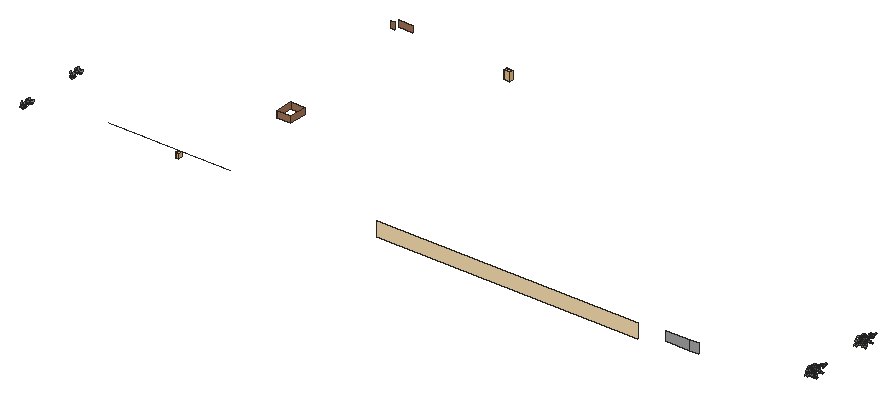
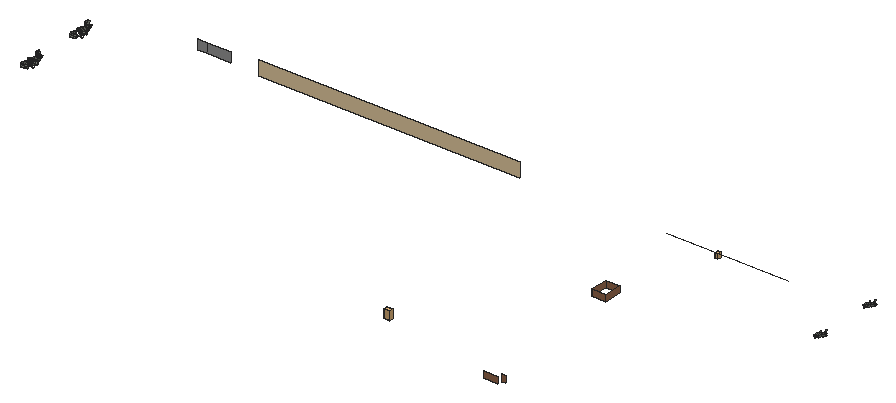
# SketchUp Ruby script. Lengths in inches.
U = 1.inch
M = Sketchup.active_model
def pt(a) = Geom::Point3d.new(a.map { |v| v * U })
def face(e, loops, mat)
  f = e.add_face(loops[0].map { |a| pt(a) })
  loops[1..].each { |l| e.add_face(l.map { |a| pt(a) }).erase! }
  f.material = f.back_material = mat if mat
  f
end
# faces: each face lists its corners as indices into pts; further lists are holes
def faces(e, pts, list, mat = nil) = list.each { |f| face(e, (f[0].is_a?(Array) ? f : [f]).map { |l| l.map { |i| pts[i] } }, mat) }
# xy, xz, yz: faces in a plane at the given z, y or x. An outline is a flat list of corners, or four numbers for a rectangle; further outlines are holes
def ring(l) = l.size == 4 ? [[l[0], l[1]], [l[2], l[1]], [l[2], l[3]], [l[0], l[3]]] : l.each_slice(2).to_a
def flat(e, list, mat, &to3) = list.each { |f| face(e, (f[0].is_a?(Array) ? f : [f]).map { |l| ring(l).map { |u, v| to3.(u, v) } }, mat) }
def xy(e, z, list, mat = nil) = flat(e, list, mat) { |x, y| [x, y, z] }
def xz(e, y, list, mat = nil) = flat(e, list, mat) { |x, z| [x, y, z] }
def yz(e, x, list, mat = nil) = flat(e, list, mat) { |y, z| [x, y, z] }
def lines(e, pts, list) = list.each { |a, b| e.add_line(pt(pts[a]), pt(pts[b])) }
# prism: a flat outline (further loops are holes) pulled along v
def prism(e, loops, v, mat = nil)
  f = face(e, loops, mat); d = Geom::Vector3d.new(v.map { |x| x * U })
  f.pushpull(f.normal.samedirection?(d) ? d.length : -d.length)
end
def box(e, o, s, mat = nil) = prism(e, [[o, [o[0] + s[0], o[1], o[2]], [o[0] + s[0], o[1] + s[1], o[2]], [o[0], o[1] + s[1], o[2]]]], [0, 0, s[2]], mat)
def at(x, y, z, deg = 0) = Geom::Transformation.translation(pt([x, y, z])) * Geom::Transformation.rotation(ORIGIN, Z_AXIS, deg.degrees)
def axes(o, x, y, z) = Geom::Transformation.new([*x, 0, *y, 0, *z, 0, *pt(o).to_a, 1])
def part(name) = M.definitions.add(name)
# library, detail: a bought-in or finely detailed component or shape, given as its bounding box
def library(name, o, s) = part(name).tap { |d| box(d.entities, o, s) }
def detail(e, o, s) = box(e.add_group.entities, o, s)
def put(e, d, t, mat = nil) = e.add_instance(d, t).tap { |i| i.material = mat if mat }
def group(e, t, mat = nil) = e.add_group.tap { |g| g.transformation = t; g.material = mat if mat }.entities
root = M.entities
M.materials.add("Material \#1").color = [140, 140, 140]
M.materials.add("[0032_Moccasin]").color = [255, 228, 181]
M.materials.add("[0132_LightGray]").color = [169, 169, 169]
M.materials.add("[Tile Ceramic Multi]").color = [165, 115, 84]
M.materials.add("viburnumblaasdfas0df1w06d").color = [98, 102, 84]
M.materials.add("viburnumbladsadfasdfad0w122").color = [125, 129, 119]
c1 = part("Component\#315")
p = [[0.25,0,0],[2.05,0.01,0.35],[1.81,4.2,1.66],[0,4.19,1.3125]]
faces(c1.entities,p,[[0,1,2,3]],"viburnumbladsadfasdfad0w122")
c2 = part("viburnumblad2")
put(c2.entities,c1,axes([-19.23,-4.49,-32.18],[83.35428,0,0],[0,79.38502,0],[0,0,83.35428]))
c3 = library("Lamp Wall Outdoor 94-02",[-1.89,-4.65,-3.17],[3.78,4.65,6.35])
c4 = library("3DGeom~3_Defintion",[-83.33,-500,-350],[620.1,1000,533.33])
c5 = part("Component\#314")
p = [[0.14,0,0],[2.58,0.05,0.25],[2.44,5.11,2.64],[0,5.05,2.39]]
faces(c5.entities,p,[[0,1,2,3]],"viburnumblaasdfas0df1w06d")
c6 = part("viburnumblad1\#2")
put(c6.entities,c5,axes([-37.25,6.23,19.31],[75.98784,0,0],[0,65.50676,0],[0,0,75.98784]))
xz(root,218.9375,[[1678.9375,30,2004.71,47.68]],"[0032_Moccasin]")
xz(root,223.9375,[[2036.3125,36,2065.6875,48]],"[0132_LightGray]")
xz(root,340.22,[[1457.08,32,1474.64,40]],"[Tile Ceramic Multi]")
xz(root,362.07,[[1457.08,32,1474.64,40]],"[Tile Ceramic Multi]")
xz(root,529.35,[[1590.92,39.28,1590.76,39.29,1590.92,39.29],[1590.92,39.28,1590.92,39.29,1591.07,39.31],[1590.92,39.28,1591.07,39.31,1591.08,39.29],[1590.76,39.29,1590.62,39.33,1590.77,39.31],[1590.76,39.29,1590.77,39.31,1590.92,39.29],
  [1591.08,39.29,1591.07,39.31,1591.22,39.34],[1591.08,39.29,1591.22,39.34,1591.23,39.33],[1590.77,39.31,1590.62,39.33,1590.62,39.34],[1590.62,39.33,1590.48,39.39,1590.62,39.34],[1591.23,39.33,1591.22,39.34,1591.35,39.4],
  [1591.23,39.33,1591.35,39.4,1591.36,39.39],[1590.62,39.34,1590.48,39.39,1590.49,39.4],[1590.48,39.39,1590.36,39.46,1590.49,39.4],[1591.36,39.39,1591.35,39.4,1591.47,39.47],[1591.36,39.39,1591.47,39.47,1591.48,39.46],
  [1590.49,39.4,1590.36,39.46,1590.37,39.47],[1590.36,39.46,1590.25,39.56,1590.37,39.47],[1591.48,39.46,1591.47,39.47,1591.58,39.57],[1591.48,39.46,1591.58,39.57,1591.59,39.56],[1590.37,39.47,1590.25,39.56,1590.26,39.57],
  [1590.87,39.49,1590.82,39.5,1590.87,39.51],[1590.87,39.49,1590.87,39.51,1590.92,39.5],[1590.87,39.49,1590.92,39.5,1590.92,39.49],[1590.92,39.49,1590.92,39.5,1590.97,39.51],[1590.92,39.49,1590.97,39.51,1590.97,39.49],
  [1590.97,39.49,1590.97,39.51,1591.02,39.52],[1590.97,39.49,1591.02,39.52,1591.02,39.5],[1590.82,39.5,1590.77,39.52,1590.82,39.52],[1590.82,39.5,1590.82,39.52,1590.87,39.51],[1591.02,39.5,1591.02,39.52,1591.06,39.54],
  [1591.02,39.5,1591.06,39.54,1591.07,39.52],[1590.77,39.52,1590.73,39.55,1590.78,39.54],[1590.77,39.52,1590.78,39.54,1590.82,39.52],[1591.07,39.52,1591.06,39.54,1591.1,39.56],[1591.07,39.52,1591.1,39.56,1591.11,39.55]],"Material \#1")
xz(root,531.36,[[1590.92,39.28,1590.92,39.29,1590.76,39.29],[1590.92,39.28,1591.07,39.31,1590.92,39.29],[1590.92,39.28,1591.08,39.29,1591.07,39.31],[1590.76,39.29,1590.77,39.31,1590.62,39.33],[1590.76,39.29,1590.92,39.29,1590.77,39.31],
  [1591.08,39.29,1591.22,39.34,1591.07,39.31],[1591.08,39.29,1591.23,39.33,1591.22,39.34],[1590.77,39.31,1590.62,39.34,1590.62,39.33],[1590.62,39.33,1590.62,39.34,1590.48,39.39],[1591.23,39.33,1591.35,39.4,1591.22,39.34],
  [1591.23,39.33,1591.36,39.39,1591.35,39.4],[1590.62,39.34,1590.49,39.4,1590.48,39.39],[1590.48,39.39,1590.49,39.4,1590.36,39.46],[1591.36,39.39,1591.47,39.47,1591.35,39.4],[1591.36,39.39,1591.48,39.46,1591.47,39.47],
  [1590.49,39.4,1590.37,39.47,1590.36,39.46],[1590.36,39.46,1590.37,39.47,1590.25,39.56],[1591.48,39.46,1591.58,39.57,1591.47,39.47],[1591.48,39.46,1591.59,39.56,1591.58,39.57],[1590.37,39.47,1590.26,39.57,1590.25,39.56],
  [1590.87,39.49,1590.87,39.51,1590.82,39.5],[1590.87,39.49,1590.92,39.49,1590.92,39.5],[1590.87,39.49,1590.92,39.5,1590.87,39.51],[1590.92,39.49,1590.97,39.49,1590.97,39.51],[1590.92,39.49,1590.97,39.51,1590.92,39.5],
  [1590.97,39.49,1591.02,39.5,1591.02,39.52],[1590.97,39.49,1591.02,39.52,1590.97,39.51],[1590.82,39.5,1590.82,39.52,1590.77,39.52],[1590.82,39.5,1590.87,39.51,1590.82,39.52],[1591.02,39.5,1591.06,39.54,1591.02,39.52],
  [1591.02,39.5,1591.07,39.52,1591.06,39.54],[1590.77,39.52,1590.78,39.54,1590.73,39.55],[1590.77,39.52,1590.82,39.52,1590.78,39.54]],"Material \#1")
xz(root,549.6875,[[1431.3125,32,1437.22,40]],"[Tile Ceramic Multi]")
xz(root,555,[[1437.22,32,1454.9375,40]],"[Tile Ceramic Multi]")
yz(root,1457.08,[[340.22,32,362.07,40]],"[Tile Ceramic Multi]")
yz(root,1474.64,[[340.22,32,362.07,40]],"[Tile Ceramic Multi]")
p = [[2065.6875,223.9375,48],[2065.6875,223.9375,36],[2076.625,224.21,36],[2076.625,224.21,48],[1491.42,223.9375,36],[1338.625,223.9375,36]]
faces(root,p,[[0,1,2,3]],"[0132_LightGray]")
lines(root,p,[[4,5]])
put(root,c2,axes([1246.61,280.32,31.73],[0.00136,-0.01101,-0.00167],[0.00866,0.00241,-0.00886],[0.00838,-0.00019,0.00814]))
put(root,c2,axes([1246.61,203.43,31.73],[0.00136,-0.01101,-0.00167],[0.00866,0.00241,-0.00886],[0.00838,-0.00019,0.00814]))
put(root,c2,axes([1248.83,286.96,33.1875],[0.0051,0.01038,-0.00415],[-0.00633,0.00571,0.00604],[0.00802,-0.00053,0.00751]))
put(root,c2,axes([1248.83,210.08,33.1875],[0.0051,0.01038,-0.00415],[-0.00633,0.00571,0.00604],[0.00802,-0.00053,0.00751]))
put(root,c2,axes([1249.1,278.54,33.3],[-0.00142,0.01147,0.00174],[-0.00575,-0.00222,0.00993],[0.01007,0.00035,0.00591]))
put(root,c2,axes([1249.1,201.66,33.3],[-0.00142,0.01147,0.00174],[-0.00575,-0.00222,0.00993],[0.01007,0.00035,0.00591]))
put(root,c2,axes([1247.41,280.15,33.05],[0.00591,-0.00652,-0.00769],[0.005,0.00963,-0.00433],[0.00875,-0.0011,0.00766]))
put(root,c2,axes([1247.41,203.27,33.05],[0.00591,-0.00652,-0.00769],[0.005,0.00963,-0.00433],[0.00875,-0.0011,0.00766]))
put(root,c2,axes([1249.99,287.16,32.28],[-0.00764,0.00611,0.00552],[-0.0043,-0.01063,0.00535],[0.00765,0.00146,0.00773]))
put(root,c2,axes([1249.99,210.27,32.28],[-0.00764,0.00611,0.00552],[-0.0043,-0.01063,0.00535],[0.00765,0.00146,0.00773]))
put(root,c2,axes([1250.43,286.67,33.61],[-0.00217,0.01153,0.00126],[-0.00855,-0.00261,0.00823],[0.00816,0.00055,0.00738]))
put(root,c2,axes([1250.43,209.78,33.61],[-0.00217,0.01153,0.00126],[-0.00855,-0.00261,0.00823],[0.00816,0.00055,0.00738]))
put(root,c2,axes([1248.45,279.5625,34.14],[0.00693,0.00224,-0.00913],[-0.00028,0.01139,0.00259],[0.0094,-0.00132,0.00681]))
put(root,c2,axes([1248.45,202.68,34.14],[0.00693,0.00224,-0.00913],[-0.00028,0.01139,0.00259],[0.0094,-0.00132,0.00681]))
put(root,c2,axes([1248.19,280.29,31.99],[-0.0039,-0.00969,0.00523],[0.00734,-0.00679,-0.00711],[0.00851,0.00087,0.00796]))
put(root,c2,axes([1248.19,203.41,31.99],[-0.0039,-0.00969,0.00523],[0.00734,-0.00679,-0.00711],[0.00851,0.00087,0.00796]))
put(root,c2,axes([1249.72,279.61,32.48],[-0.00693,-0.00224,0.00913],[0.00254,-0.01137,-0.00086],[0.00905,0.00148,0.00724]))
put(root,c2,axes([1249.72,202.73,32.48],[-0.00693,-0.00224,0.00913],[0.00254,-0.01137,-0.00086],[0.00905,0.00148,0.00724]))
put(root,c2,axes([1249.4375,287.32,34.32],[0.00908,0.00254,-0.00688],[-0.00118,0.01053,0.00207],[0.00732,-0.00116,0.00806]))
put(root,c2,axes([1249.4375,210.4375,34.32],[0.00908,0.00254,-0.00688],[-0.00118,0.01053,0.00207],[0.00732,-0.00116,0.00806]))
put(root,c2,axes([1250.64,286.79,35.2],[0.00489,0.00995,-0.00397],[-0.00703,0.00634,0.00672],[0.00802,-0.00053,0.00751]))
put(root,c2,axes([1250.64,209.91,35.2],[0.00489,0.00995,-0.00397],[-0.00703,0.00634,0.00672],[0.00802,-0.00053,0.00751]))
put(root,c2,axes([1248.78,288.22,33.3],[0.00664,-0.00572,-0.00612],[0.00571,0.0099,-0.00294],[0.00728,-0.00165,0.00803]))
put(root,c2,axes([1248.78,211.34,33.3],[0.00664,-0.00572,-0.00612],[0.00571,0.0099,-0.00294],[0.00728,-0.00165,0.00803]))
put(root,c2,axes([1249.06,280.63,33.33],[0.00142,-0.01147,-0.00174],[0.00801,0.00224,-0.0082],[0.00838,-0.00019,0.00814]))
put(root,c2,axes([1249.06,203.75,33.33],[0.00142,-0.01147,-0.00174],[0.00801,0.00224,-0.0082],[0.00838,-0.00019,0.00814]))
put(root,c2,axes([1251.82,286.86,34.32],[-0.00796,0.00636,0.00575],[-0.00398,-0.00984,0.00495],[0.00765,0.00146,0.00773]))
put(root,c2,axes([1251.82,209.98,34.32],[-0.00796,0.00636,0.00575],[-0.00398,-0.00984,0.00495],[0.00765,0.00146,0.00773]))
put(root,c2,axes([1251.07,287.73,33.13],[-0.00908,-0.00254,0.00688],[0.00302,-0.01141,-0.00024],[0.00679,0.00165,0.00837]))
put(root,c2,axes([1251.07,210.84,33.13],[-0.00908,-0.00254,0.00688],[0.00302,-0.01141,-0.00024],[0.00679,0.00165,0.00837]))
put(root,c2,axes([1250.15,288.72,33.78],[0.00217,-0.01153,-0.00126],[0.00998,0.00257,-0.00587],[0.00594,-0.00007,0.00905]))
put(root,c2,axes([1250.15,211.84,33.78],[0.00217,-0.01153,-0.00126],[0.00998,0.00257,-0.00587],[0.00594,-0.00007,0.00905]))
put(root,c2,axes([1250.57,288.28,35.21],[0.00796,-0.00636,-0.00575],[0.00571,0.0099,-0.00294],[0.00646,-0.00097,0.0087]))
put(root,c2,axes([1250.57,211.4,35.21],[0.00796,-0.00636,-0.00575],[0.00571,0.0099,-0.00294],[0.00646,-0.00097,0.0087]))
put(root,c2,axes([1251.75,288.35,34.33],[-0.00489,-0.00995,0.00397],[0.00876,-0.00628,-0.0047],[0.00608,0.00102,0.00892]))
put(root,c2,axes([1251.75,211.47,34.33],[-0.00489,-0.00995,0.00397],[0.00876,-0.00628,-0.0047],[0.00608,0.00102,0.00892]))
put(root,c3,at(1428.92,223.9375,32.6))
put(root,c4,axes([1590.92,531.05,44.51],[0.012,0,0],[0,0,0.01068],[0,0.00833,0]),"Material \#1")
put(root,c2,axes([2183.65,344.92,39.97],[-0.00351,0.01047,-0.00368],[-0.0097,-0.00494,-0.00456],[-0.00545,0.00224,0.00858]))
put(root,c2,axes([2183.65,268.04,39.97],[-0.00351,0.01047,-0.00368],[-0.0097,-0.00494,-0.00456],[-0.00545,0.00224,0.00858]))
put(root,c2,axes([2182.64,345.63,39.1875],[0.00896,0.00518,0.00557],[-0.00429,0.01059,-0.00268],[-0.00611,0.00033,0.00835]))
put(root,c2,axes([2182.64,268.75,39.1875],[0.00896,0.00518,0.00557],[-0.00429,0.01059,-0.00268],[-0.00611,0.00033,0.00835]))
put(root,c2,axes([2183.85,344.63,38.53],[0.00385,0.01107,0.00134],[-0.00965,0.00395,-0.00558],[-0.00546,0.00115,0.0087]))
put(root,c2,axes([2183.85,267.75,38.53],[0.00385,0.01107,0.00134],[-0.00965,0.00395,-0.00558],[-0.00546,0.00115,0.0087]))
put(root,c2,axes([2185.31,344.47,38.125],[-0.00267,0.00936,-0.00422],[-0.0097,-0.00494,-0.00456],[-0.00579,0.00336,0.00814]))
put(root,c2,axes([2185.31,267.59,38.125],[-0.00267,0.00936,-0.00422],[-0.0097,-0.00494,-0.00456],[-0.00579,0.00336,0.00814]))
put(root,c2,axes([2185.14,345.36,39.29],[-0.00882,0.00375,-0.00654],[-0.00425,-0.0099,-0.00033],[-0.00607,0.00296,0.00807]))
put(root,c2,axes([2185.14,268.48,39.29],[-0.00882,0.00375,-0.00654],[-0.00425,-0.0099,-0.00033],[-0.00607,0.00296,0.00807]))
put(root,c2,axes([2184.32,346.22,40.28],[-0.00896,-0.00518,-0.00557],[0.00268,-0.0102,0.00462],[-0.00697,0.00288,0.00746]))
put(root,c2,axes([2184.32,269.34,40.28],[-0.00896,-0.00518,-0.00557],[0.00268,-0.0102,0.00462],[-0.00697,0.00288,0.00746]))
put(root,c2,axes([2183.58,346.0625,38.17],[0.00882,-0.00375,0.00654],[0.00302,0.01118,0.0023],[-0.00701,0.00026,0.00774]))
put(root,c2,axes([2183.58,269.18,38.17],[0.00882,-0.00375,0.00654],[0.00302,0.01118,0.0023],[-0.00701,0.00026,0.00774]))
put(root,c2,axes([2183.31,346.93,39.49],[0.00351,-0.01047,0.00368],[0.00809,0.00534,0.0065],[-0.00763,0.00098,0.00722]))
put(root,c2,axes([2183.31,270.04,39.49],[0.00351,-0.01047,0.00368],[0.00809,0.00534,0.0065],[-0.00763,0.00098,0.00722]))
put(root,c2,axes([2185.88,345.59,38.29],[-0.00935,-0.0054,-0.00582],[0.00241,-0.00918,0.00416],[-0.00697,0.00288,0.00746]))
put(root,c2,axes([2185.88,268.71,38.29],[-0.00935,-0.0054,-0.00582],[0.00241,-0.00918,0.00416],[-0.00697,0.00288,0.00746]))
put(root,c2,axes([2184.64,346.54,38.82],[-0.00385,-0.01107,-0.00134],[0.00835,-0.0037,0.00784],[-0.00761,0.00206,0.00711]))
put(root,c2,axes([2184.64,269.66,38.82],[-0.00385,-0.01107,-0.00134],[0.00835,-0.0037,0.00784],[-0.00761,0.00206,0.00711]))
put(root,c2,axes([2187.57,333.39,39.18],[0.00449,0.0055,0.01006],[-0.01013,0.00737,0.00027],[-0.00579,-0.00855,0.00654]))
put(root,c2,axes([2187.57,256.51,39.18],[0.00449,0.0055,0.01006],[-0.01013,0.00737,0.00027],[-0.00579,-0.00855,0.00654]))
put(root,c2,axes([2184.83,346.18,37.45],[0.00337,-0.01006,0.00353],[0.00874,0.00576,0.00702],[-0.00763,0.00098,0.00722]))
put(root,c2,axes([2184.83,269.3,37.45],[0.00337,-0.01006,0.00353],[0.00874,0.00576,0.00702],[-0.00763,0.00098,0.00722]))
put(root,c2,axes([2188.24,356.2,38.47],[-0.00103,0.00921,-0.00523],[-0.01005,-0.00269,-0.00267],[-0.00353,0.00478,0.00792]))
put(root,c2,axes([2188.24,279.32,38.47],[-0.00103,0.00921,-0.00523],[-0.01005,-0.00269,-0.00267],[-0.00353,0.00478,0.00792]))
put(root,c6,axes([2189.82,342.8,33.29],[-0.00628,0.01217,-0.00276],[-0.013,-0.00799,-0.00559],[-0.00514,0.00045,0.01101]))
put(root,c6,axes([2189.82,265.92,33.29],[-0.00628,0.01217,-0.00276],[-0.013,-0.00799,-0.00559],[-0.00514,0.00045,0.01101]))
put(root,c2,axes([2189.24,333.99,38.72],[-0.00344,0.0098,0.00674],[-0.01109,0.00113,-0.00697],[-0.00574,-0.00778,0.00739]))
put(root,c2,axes([2189.24,257.11,38.72],[-0.00344,0.0098,0.00674],[-0.01109,0.00113,-0.00697],[-0.00574,-0.00778,0.00739]))
put(root,c2,axes([2188.86,332.93,39.97],[-0.00935,0.00836,-0.00053],[-0.00531,-0.00639,-0.00919],[-0.00638,-0.00686,0.0077]))
put(root,c2,axes([2188.86,256.05,39.97],[-0.00935,0.00836,-0.00053],[-0.00531,-0.00639,-0.00919],[-0.00638,-0.00686,0.0077]))
put(root,c2,axes([2188.23,355.64,37.17],[0.00602,0.00882,-0.00114],[-0.00807,0.00476,-0.00535],[-0.00378,0.00387,0.00824]))
put(root,c2,axes([2188.23,278.76,37.17],[0.00602,0.00882,-0.00114],[-0.00807,0.00476,-0.00535],[-0.00378,0.00387,0.00824]))
put(root,c6,axes([2187.39,345.72,36.11],[-0.0079,-0.01009,-0.00146],[0.00852,-0.00752,0.00905],[-0.00687,0.00486,0.00819]))
put(root,c6,axes([2187.39,268.84,36.11],[-0.0079,-0.01009,-0.00146],[0.00852,-0.00752,0.00905],[-0.00687,0.00486,0.00819]))
put(root,c2,axes([2189.43,355.08,36.73],[-0.00059,0.00795,-0.00557],[-0.01005,-0.00269,-0.00267],[-0.00362,0.00574,0.0073]))
put(root,c2,axes([2189.43,278.2,36.73],[-0.00059,0.00795,-0.00557],[-0.01005,-0.00269,-0.00267],[-0.00362,0.00574,0.0073]))
put(root,c6,axes([2189.1,344.47,35.23],[-0.01179,-0.00065,-0.00527],[-0.00088,-0.01435,0.00336],[-0.0049,0.00375,0.00968]))
put(root,c6,axes([2189.1,267.58,35.23],[-0.01179,-0.00065,-0.00527],[-0.00088,-0.01435,0.00336],[-0.0049,0.00375,0.00968]))
put(root,c2,axes([2187.44,356.91,37.67],[0.00954,0.00326,0.00362],[-0.0016,0.00968,-0.00428],[-0.00457,0.00326,0.00811]))
put(root,c2,axes([2187.44,280.03,37.67],[0.00954,0.00326,0.00362],[-0.0016,0.00968,-0.00428],[-0.00457,0.00326,0.00811]))
put(root,c2,axes([2189.21,335.46,37.7],[0.00469,0.00575,0.0105],[-0.00912,0.00663,0.00024],[-0.00579,-0.00855,0.00654]))
put(root,c2,axes([2189.21,258.58,37.7],[0.00469,0.00575,0.0105],[-0.00912,0.00663,0.00024],[-0.00579,-0.00855,0.00654]))
put(root,c2,axes([2188.11,334.93,38.55],[0.00979,-0.00202,0.00749],[-0.00391,0.00808,0.00687],[-0.00651,-0.00873,0.00566]))
put(root,c2,axes([2188.11,258.05,38.55],[0.00979,-0.00202,0.00749],[-0.00391,0.00808,0.00687],[-0.00651,-0.00873,0.00566]))
put(root,c2,axes([2189.59,356.09,37.66],[-0.00747,0.00421,-0.00626],[-0.00602,-0.00754,0.00188],[-0.00396,0.00545,0.00734]))
put(root,c2,axes([2189.59,279.21,37.66],[-0.00747,0.00421,-0.00626],[-0.00602,-0.00754,0.00188],[-0.00396,0.00545,0.00734]))
put(root,c2,axes([2188.99,345.19,39.72],[0.00608,0.00542,0.00802],[-0.00721,0.00886,-0.00053],[-0.00646,-0.00478,0.00813]))
put(root,c2,axes([2188.99,268.3,39.72],[0.00608,0.00542,0.00802],[-0.00721,0.00886,-0.00053],[-0.00646,-0.00478,0.00813]))
put(root,c6,axes([2191.43,336.95,36.05],[-0.00239,0.00794,0.01052],[-0.01424,0.00397,-0.00606],[-0.00563,-0.01073,0.00596]))
put(root,c6,axes([2191.43,260.07,36.05],[-0.00239,0.00794,0.01052],[-0.01424,0.00397,-0.00606],[-0.00563,-0.01073,0.00596]))
put(root,c2,axes([2190.09,344.61,40.46],[-0.00637,0.00937,-0.00151],[-0.00692,-0.00583,-0.00699],[-0.0065,-0.00298,0.00892]))
put(root,c2,axes([2190.09,267.73,40.46],[-0.00637,0.00937,-0.00151],[-0.00692,-0.00583,-0.00699],[-0.0065,-0.00298,0.00892]))
put(root,c2,axes([2189.15,357.2,38.46],[-0.00954,-0.00326,-0.00362],[0.00044,-0.00861,0.00611],[-0.00482,0.0055,0.00684]))
put(root,c2,axes([2189.15,280.32,38.46],[-0.00954,-0.00326,-0.00362],[0.00044,-0.00861,0.00611],[-0.00482,0.0055,0.00684]))
put(root,c2,axes([2190.6,342.7,32],[-0.00442,0.0106,-0.0025],[-0.00963,-0.00512,-0.00451],[-0.00488,0.00074,0.00902]))
put(root,c2,axes([2190.6,265.82,32],[-0.00442,0.0106,-0.0025],[-0.00963,-0.00512,-0.00451],[-0.00488,0.00074,0.00902]))
put(root,c2,axes([2190.5625,345.21,39.0625],[-0.00021,0.01046,0.0046],[-0.01011,0.00244,-0.006],[-0.00617,-0.00398,0.00877]))
put(root,c2,axes([2190.5625,268.33,39.0625],[-0.00021,0.01046,0.0046],[-0.01011,0.00244,-0.006],[-0.00617,-0.00398,0.00877]))
put(root,c2,axes([2190.51,335.13,38.55],[-0.00898,0.00802,-0.00051],[-0.00573,-0.0069,-0.00993],[-0.00638,-0.00686,0.0077]))
put(root,c2,axes([2190.51,258.25,38.55],[-0.00898,0.00802,-0.00051],[-0.00573,-0.0069,-0.00993],[-0.00638,-0.00686,0.0077]))
put(root,c2,axes([2189.49,343.42,31.34],[0.00896,0.00518,0.00557],[-0.00512,0.01053,-0.00146],[-0.00544,-0.00118,0.00865]))
put(root,c2,axes([2189.49,266.53,31.34],[0.00896,0.00518,0.00557],[-0.00512,0.01053,-0.00146],[-0.00544,-0.00118,0.00865]))
put(root,c2,axes([2190.71,342.6,30.53],[0.00321,0.01115,0.00217],[-0.01022,0.00386,-0.00469],[-0.00482,-0.00036,0.00904]))
put(root,c2,axes([2190.71,265.72,30.53],[0.00321,0.01115,0.00217],[-0.01022,0.00386,-0.00469],[-0.00482,-0.00036,0.00904]))
put(root,c6,axes([2191.58,339.02,34.64],[0.00666,0.0005,0.01169],[-0.01037,0.01092,0.00488],[-0.00799,-0.01005,0.00435]))
put(root,c6,axes([2191.58,262.14,34.64],[0.00666,0.0005,0.01169],[-0.01037,0.01092,0.00488],[-0.00799,-0.01005,0.00435]))
put(root,c2,axes([2189.83,334.52,39.87],[-0.00979,0.00202,-0.00749],[0.00256,-0.01065,-0.00589],[-0.00735,-0.00634,0.0073]))
put(root,c2,axes([2189.83,257.63,39.87],[-0.00979,0.00202,-0.00749],[0.00256,-0.01065,-0.00589],[-0.00735,-0.00634,0.0073]))
put(root,c2,axes([2188.64,334.11,40.97],[-0.00449,-0.0055,-0.01006],[0.00843,-0.00922,0.00132],[-0.00807,-0.00651,0.00641]))
put(root,c2,axes([2188.64,257.22,40.97],[-0.00449,-0.0055,-0.01006],[0.00843,-0.00922,0.00132],[-0.00807,-0.00651,0.00641]))
put(root,c2,axes([2190.21,355.93,36.63],[-0.00996,-0.0034,-0.00378],[0.0004,-0.00774,0.0055],[-0.00482,0.0055,0.00684]))
put(root,c2,axes([2190.21,279.05,36.63],[-0.00996,-0.0034,-0.00378],[0.0004,-0.00774,0.0055],[-0.00482,0.0055,0.00684]))
put(root,c2,axes([2188.28,356.875,36.58],[0.00747,-0.00421,0.00626],[0.0054,0.00929,-0.00022],[-0.00543,0.00331,0.00761]))
put(root,c2,axes([2188.28,279.99,36.58],[0.00747,-0.00421,0.00626],[0.0054,0.00929,-0.00022],[-0.00543,0.00331,0.00761]))
put(root,c6,axes([2192.59,351.68,32.26],[-0.00299,0.01151,-0.00453],[-0.01374,-0.0047,-0.00282],[-0.00346,0.0036,0.01051]))
put(root,c6,axes([2192.59,274.8,32.26],[-0.00299,0.01151,-0.00453],[-0.01374,-0.0047,-0.00282],[-0.00346,0.0036,0.01051]))
put(root,c2,axes([2188.35,357.92,37.66],[0.00103,-0.00921,0.00523],[0.0089,0.00377,0.00451],[-0.00586,0.00398,0.00703]))
put(root,c2,axes([2188.35,281.04,37.66],[0.00103,-0.00921,0.00523],[0.0089,0.00377,0.00451],[-0.00586,0.00398,0.00703]))
put(root,c2,axes([2188.92,336.43,38.57],[0.0093,-0.00683,-0.00004],[0.0036,0.00454,0.01078],[-0.00642,-0.00906,0.00528]))
put(root,c2,axes([2188.92,259.54,38.57],[0.0093,-0.00683,-0.00004],[0.0036,0.00454,0.01078],[-0.00642,-0.00906,0.00528]))
put(root,c2,axes([2190.78,346.3,37.83],[0.00634,0.00566,0.00838],[-0.00649,0.00797,-0.00047],[-0.00646,-0.00478,0.00813]))
put(root,c2,axes([2190.78,269.42,37.83],[0.00634,0.00566,0.00838],[-0.00649,0.00797,-0.00047],[-0.00646,-0.00478,0.00813]))
put(root,c2,axes([2189.77,346.26,38.8],[0.0088,-0.00279,0.00674],[-0.001,0.00912,0.00509],[-0.00721,-0.00491,0.00738]))
put(root,c2,axes([2189.77,269.38,38.8],[0.0088,-0.00279,0.00674],[-0.001,0.00912,0.00509],[-0.00721,-0.00491,0.00738]))
put(root,c2,axes([2189.37,357.14,37.02],[-0.00602,-0.00882,0.00114],[0.00718,-0.00382,0.00749],[-0.0056,0.00489,0.00671]))
put(root,c2,axes([2189.37,280.26,37.02],[-0.00602,-0.00882,0.00114],[0.00718,-0.00382,0.00749],[-0.0056,0.00489,0.00671]))
put(root,c6,axes([2192.93,346.75,35.87],[0.00062,0.00927,0.00842],[-0.01215,0.00581,-0.0055],[-0.00687,-0.00679,0.00799]))
put(root,c6,axes([2192.93,269.86,35.87],[0.00062,0.00927,0.00842],[-0.01215,0.00581,-0.0055],[-0.00687,-0.00679,0.00799]))
put(root,c2,axes([2191.92,345.85,38.61],[-0.00611,0.009,-0.00145],[-0.00747,-0.0063,-0.00755],[-0.0065,-0.00298,0.00892]))
put(root,c2,axes([2191.92,268.97,38.61],[-0.00611,0.009,-0.00145],[-0.00747,-0.0063,-0.00755],[-0.0065,-0.00298,0.00892]))
put(root,c2,axes([2188.73,335.68,39.99],[0.00344,-0.0098,-0.00674],[0.00895,-0.00296,0.00831],[-0.00812,-0.00729,0.00557]))
put(root,c2,axes([2188.73,258.8,39.99],[0.00344,-0.0098,-0.00674],[0.00895,-0.00296,0.00831],[-0.00812,-0.00729,0.00557]))
